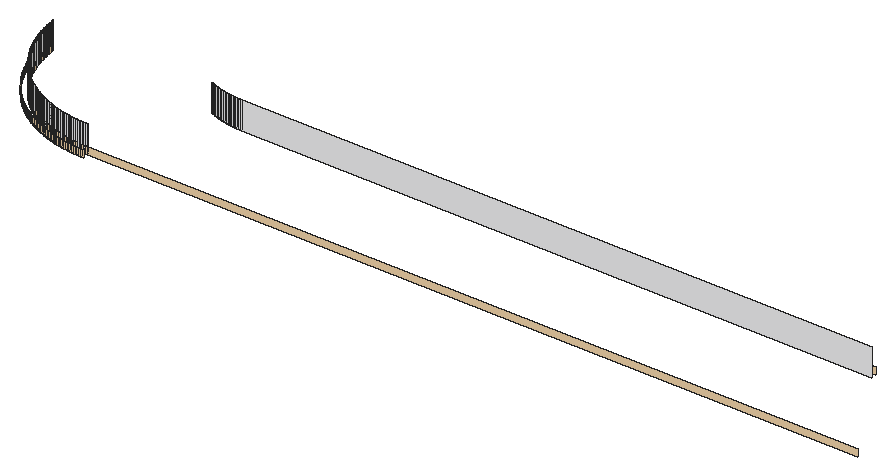
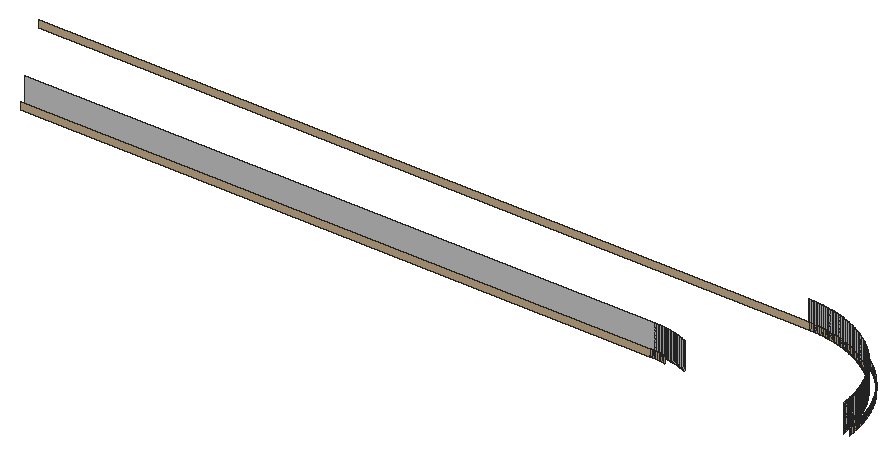
# SketchUp Ruby script. Lengths in inches.
U = 1.inch
M = Sketchup.active_model
def pt(a) = Geom::Point3d.new(a.map { |v| v * U })
def face(e, loops, mat)
  f = e.add_face(loops[0].map { |a| pt(a) })
  loops[1..].each { |l| e.add_face(l.map { |a| pt(a) }).erase! }
  f.material = f.back_material = mat if mat
  f
end
# faces: each face lists its corners as indices into pts; further lists are holes
def faces(e, pts, list, mat = nil) = list.each { |f| face(e, (f[0].is_a?(Array) ? f : [f]).map { |l| l.map { |i| pts[i] } }, mat) }
# xy, xz, yz: faces in a plane at the given z, y or x. An outline is a flat list of corners, or four numbers for a rectangle; further outlines are holes
def ring(l) = l.size == 4 ? [[l[0], l[1]], [l[2], l[1]], [l[2], l[3]], [l[0], l[3]]] : l.each_slice(2).to_a
def flat(e, list, mat, &to3) = list.each { |f| face(e, (f[0].is_a?(Array) ? f : [f]).map { |l| ring(l).map { |u, v| to3.(u, v) } }, mat) }
def xy(e, z, list, mat = nil) = flat(e, list, mat) { |x, y| [x, y, z] }
def xz(e, y, list, mat = nil) = flat(e, list, mat) { |x, z| [x, y, z] }
def yz(e, x, list, mat = nil) = flat(e, list, mat) { |y, z| [x, y, z] }
def lines(e, pts, list) = list.each { |a, b| e.add_line(pt(pts[a]), pt(pts[b])) }
# prism: a flat outline (further loops are holes) pulled along v
def prism(e, loops, v, mat = nil)
  f = face(e, loops, mat); d = Geom::Vector3d.new(v.map { |x| x * U })
  f.pushpull(f.normal.samedirection?(d) ? d.length : -d.length)
end
def box(e, o, s, mat = nil) = prism(e, [[o, [o[0] + s[0], o[1], o[2]], [o[0] + s[0], o[1] + s[1], o[2]], [o[0], o[1] + s[1], o[2]]]], [0, 0, s[2]], mat)
def at(x, y, z, deg = 0) = Geom::Transformation.translation(pt([x, y, z])) * Geom::Transformation.rotation(ORIGIN, Z_AXIS, deg.degrees)
def axes(o, x, y, z) = Geom::Transformation.new([*x, 0, *y, 0, *z, 0, *pt(o).to_a, 1])
def part(name) = M.definitions.add(name)
# library, detail: a bought-in or finely detailed component or shape, given as its bounding box
def library(name, o, s) = part(name).tap { |d| box(d.entities, o, s) }
def detail(e, o, s) = box(e.add_group.entities, o, s)
def put(e, d, t, mat = nil) = e.add_instance(d, t).tap { |i| i.material = mat if mat }
def group(e, t, mat = nil) = e.add_group.tap { |g| g.transformation = t; g.material = mat if mat }.entities
root = M.entities
M.materials.add("False Ceiling Light").color = [254, 223, 179]
M.materials.add("[Quartz Light Grey]").color = [251, 251, 252]
xz(root,43.5,[[44.53,115.32,44.76,116.49],[44.76,115.32,45,116.49]],"False Ceiling Light")
xz(root,44.5,[[44.55,115.32,44.77,116.49],[44.77,115.32,45.01,116.49],[45.01,115.32,176.99,116.49]],"False Ceiling Light")
xz(root,44.5,[[44.55,115.32,44.77,120],[44.77,115.32,45.01,120]],"[Quartz Light Grey]")
xz(root,62.5,[[56.8,115.32,56.99,120],[56.99,115.32,165.01,120]],"[Quartz Light Grey]")
xz(root,62.51,[[56.39,115.32,56.59,120]],"[Quartz Light Grey]")
xz(root,63.5,[[56.62,115.32,56.81,116.49],[56.81,115.32,56.99,116.49],[56.99,115.32,165.01,116.49]],"False Ceiling Light")
p = [[43.35,43.56,115.32],[43.59,43.54,115.32],[43.59,43.54,116.49],[43.35,43.56,116.49],[43.82,43.53,115.32],[43.82,43.53,116.49],
  [44.06,43.52,115.32],[44.06,43.52,116.49],[44.29,43.51,115.32],[44.29,43.51,116.49],[44.53,43.5,115.32],[44.53,43.5,116.49],
  [42.18,43.68,115.32],[42.41,43.65,115.32],[42.41,43.65,116.49],[42.18,43.68,116.49],[42.65,43.625,115.32],[42.65,43.625,116.49],
  [42.88,43.6,115.32],[42.88,43.6,116.49],[43.12,43.58,115.32],[43.12,43.58,116.49],[41.48,43.78,115.32],[41.71,43.74,115.32],
  [41.71,43.74,116.49],[41.48,43.78,116.49],[41.95,43.71,115.32],[41.95,43.71,116.49],[41.02,43.86,115.32],[41.25,43.82,115.32],
  [41.25,43.82,116.49],[41.02,43.86,116.49],[40.32,43.99,115.32],[40.55,43.94,115.32],[40.55,43.94,116.49],[40.32,43.99,116.49],
  [40.78,43.9,115.32],[40.78,43.9,116.49],[39.86,44.09,115.32],[40.09,44.04,115.32],[40.09,44.04,116.49],[39.86,44.09,116.49],
  [39.4,44.21,115.32],[39.63,44.15,115.32],[39.63,44.15,116.49],[39.4,44.21,116.49],[39.18,44.27,115.32],[39.18,44.27,116.49],
  [38.72,44.39,115.32],[38.95,44.33,115.32],[38.95,44.33,116.49],[38.72,44.39,116.49],[38.5,44.46,115.32],[38.5,44.46,116.49],
  [38.05,44.6,115.32],[38.27,44.53,115.32],[38.27,44.53,116.49],[38.05,44.6,116.49],[43.65,44.54,115.32],[43.43,44.56,115.32],
  [43.43,44.56,116.49],[43.65,44.54,116.49],[43.43,44.56,115.32],[43.65,44.54,115.32],[43.65,44.54,120],[43.43,44.56,120],
  [43.875,44.53,115.32],[43.875,44.53,116.49],[43.875,44.53,115.32],[43.875,44.53,120],[44.1,44.52,115.32],[44.1,44.52,116.49],
  [44.1,44.52,115.32],[44.1,44.52,120],[44.32,44.51,115.32],[44.32,44.51,116.49],[44.32,44.51,115.32],[44.32,44.51,120],
  [44.55,44.5,115.32],[44.55,44.5,116.49],[44.55,44.5,115.32],[44.55,44.5,120],[37.82,44.68,115.32],[37.82,44.68,116.49],
  [42.53,44.64,115.32],[42.31,44.67,115.32],[42.31,44.67,116.49],[42.53,44.64,116.49],[42.31,44.67,115.32],[42.53,44.64,115.32],
  [42.53,44.64,120],[42.31,44.67,120],[42.75,44.62,115.32],[42.75,44.62,116.49],[42.75,44.62,115.32],[42.75,44.62,120],
  [42.98,44.6,115.32],[42.98,44.6,116.49],[42.98,44.6,115.32],[42.98,44.6,120],[43.2,44.58,115.32],[43.2,44.58,116.49],
  [43.2,44.58,115.32],[43.2,44.58,120],[37.6,44.75,115.32],[37.6,44.75,116.49],[41.86,44.73,115.32],[41.64,44.76,115.32],
  [41.64,44.76,116.49],[41.86,44.73,116.49],[41.64,44.76,115.32],[41.86,44.73,115.32],[41.86,44.73,120],[41.64,44.76,120],
  [42.08,44.7,115.32],[42.08,44.7,116.49],[42.08,44.7,115.32],[42.08,44.7,120],[37.16,44.91,115.32],[37.38,44.83,115.32],
  [37.38,44.83,116.49],[37.16,44.91,116.49],[41.19,44.84,115.32],[40.97,44.88,115.32],[40.97,44.88,116.49],[41.19,44.84,116.49],
  [40.97,44.88,115.32],[41.19,44.84,115.32],[41.19,44.84,120],[40.97,44.88,120],[41.41,44.8,115.32],[41.41,44.8,116.49],
  [41.41,44.8,115.32],[41.41,44.8,120],[36.9375,44.99,115.32],[36.9375,44.99,116.49],[40.75,44.92,115.32],[40.53,44.97,115.32],
  [40.53,44.97,116.49],[40.75,44.92,116.49],[40.53,44.97,115.32],[40.75,44.92,115.32],[40.75,44.92,120],[40.53,44.97,120],
  [36.72,45.08,115.32],[36.72,45.08,116.49],[40.31,45.02,115.32],[40.09,45.07,115.32],[40.09,45.07,116.49],[40.31,45.02,116.49],
  [40.09,45.07,115.32],[40.31,45.02,115.32],[40.31,45.02,120],[40.09,45.07,120],[36.5,45.17,115.32],[36.5,45.17,116.49],
  [39.87,45.12,115.32],[39.65,45.18,115.32],[39.65,45.18,116.49],[39.87,45.12,116.49],[39.65,45.18,115.32],[39.87,45.12,115.32],
  [39.87,45.12,120],[39.65,45.18,120],[36.28,45.26,115.32],[36.28,45.26,116.49],[39.44,45.23,115.32],[39.22,45.29,115.32],
  [39.22,45.29,116.49],[39.44,45.23,116.49],[39.22,45.29,115.32],[39.44,45.23,115.32],[39.44,45.23,120],[39.22,45.29,120],
  [36.0625,45.35,115.32],[36.0625,45.35,116.49],[39,45.35,115.32],[39,45.35,116.49],[39,45.35,115.32],[39,45.35,120],
  [35.63,45.54,115.32],[35.85,45.45,115.32],[35.85,45.45,116.49],[35.63,45.54,116.49],[38.79,45.42,115.32],[38.57,45.48,115.32],
  [38.57,45.48,116.49],[38.79,45.42,116.49],[38.57,45.48,115.32],[38.79,45.42,115.32],[38.79,45.42,120],[38.57,45.48,120],
  [35.42,45.64,115.32],[35.42,45.64,116.49],[38.36,45.55,115.32],[38.36,45.55,116.49],[38.36,45.55,115.32],[38.36,45.55,120],
  [35.21,45.74,115.32],[35.21,45.74,116.49],[38.14,45.625,115.32],[37.93,45.7,115.32],[37.93,45.7,116.49],[38.14,45.625,116.49],
  [37.93,45.7,115.32],[38.14,45.625,115.32],[38.14,45.625,120],[37.93,45.7,120],[35,45.85,115.32],[35,45.85,116.49],
  [37.72,45.77,115.32],[37.72,45.77,116.49],[37.72,45.77,115.32],[37.72,45.77,120],[34.79,45.95,115.32],[34.79,45.95,116.49],
  [37.51,45.85,115.32],[37.3,45.93,115.32],[37.3,45.93,116.49],[37.51,45.85,116.49],[37.3,45.93,115.32],[37.51,45.85,115.32],
  [37.51,45.85,120],[37.3,45.93,120],[37.09,46.01,115.32],[37.09,46.01,116.49],[37.09,46.01,115.32],[37.09,46.01,120],
  [34.58,46.06,115.32],[34.58,46.06,116.49],[36.875,46.09,115.32],[36.875,46.09,116.49],[36.875,46.09,115.32],[36.875,46.09,120],
  [34.37,46.17,115.32],[34.37,46.17,116.49],[36.67,46.18,115.32],[36.67,46.18,116.49],[36.67,46.18,115.32],[36.67,46.18,120],
  [34.16,46.28,115.32],[34.16,46.28,116.49],[36.46,46.27,115.32],[36.46,46.27,116.49],[36.46,46.27,115.32],[36.46,46.27,120],
  [33.95,46.4,115.32],[33.95,46.4,116.49],[36.26,46.36,115.32],[36.26,46.36,116.49],[36.26,46.36,115.32],[36.26,46.36,120],
  [33.75,46.51,115.32],[33.75,46.51,116.49],[36.05,46.45,115.32],[36.05,46.45,116.49],[36.05,46.45,115.32],[36.05,46.45,120],
  [33.55,46.63,115.32],[33.55,46.63,116.49],[35.85,46.55,115.32],[35.64,46.64,115.32],[35.64,46.64,116.49],[35.85,46.55,116.49],
  [35.64,46.64,115.32],[35.85,46.55,115.32],[35.85,46.55,120],[35.64,46.64,120],[33.34,46.75,115.32],[33.34,46.75,116.49],
  [35.44,46.74,115.32],[35.44,46.74,116.49],[35.44,46.74,115.32],[35.44,46.74,120],[35.24,46.84,115.32],[35.24,46.84,116.49],
  [35.24,46.84,115.32],[35.24,46.84,120],[33.14,46.88,115.32],[33.14,46.88,116.49],[35.04,46.95,115.32],[35.04,46.95,116.49],
  [35.04,46.95,115.32],[35.04,46.95,120],[32.94,47,115.32],[32.94,47,116.49],[34.84,47.05,115.32],[34.84,47.05,116.49],
  [34.84,47.05,115.32],[34.84,47.05,120],[32.75,47.13,115.32],[32.75,47.13,116.49],[32.55,47.26,115.32],[32.55,47.26,116.49],
  [34.64,47.16,115.32],[34.64,47.16,116.49],[34.64,47.16,115.32],[34.64,47.16,120],[34.45,47.27,115.32],[34.45,47.27,116.49],
  [34.45,47.27,115.32],[34.45,47.27,120],[32.35,47.39,115.32],[32.35,47.39,116.49],[34.25,47.38,115.32],[34.25,47.38,116.49],
  [34.25,47.38,115.32],[34.25,47.38,120],[32.16,47.52,115.32],[32.16,47.52,116.49],[34.06,47.49,115.32],[34.06,47.49,116.49],
  [34.06,47.49,115.32],[34.06,47.49,120],[31.97,47.66,115.32],[31.97,47.66,116.49],[33.86,47.61,115.32],[33.86,47.61,116.49],
  [33.86,47.61,115.32],[33.86,47.61,120],[33.67,47.73,115.32],[33.67,47.73,116.49],[33.67,47.73,115.32],[33.67,47.73,120],
  [31.77,47.8,115.32],[31.77,47.8,116.49],[33.48,47.85,115.32],[33.48,47.85,116.49],[33.48,47.85,115.32],[33.48,47.85,120],
  [31.58,47.9375,115.32],[31.58,47.9375,116.49],[33.29,47.97,115.32],[33.29,47.97,116.49],[33.29,47.97,115.32],[33.29,47.97,120],
  [31.4,48.08,115.32],[31.4,48.08,116.49],[33.1,48.09,115.32],[33.1,48.09,116.49],[33.1,48.09,115.32],[33.1,48.09,120],
  [31.21,48.22,115.32],[31.21,48.22,116.49],[32.92,48.22,115.32],[32.92,48.22,116.49],[32.92,48.22,115.32],[32.92,48.22,120],
  [31.02,48.37,115.32],[31.02,48.37,116.49],[32.73,48.35,115.32],[32.73,48.35,116.49],[32.73,48.35,115.32],[32.73,48.35,120],
  [32.55,48.47,115.32],[32.55,48.47,116.49],[32.55,48.47,115.32],[32.55,48.47,120],[30.84,48.51,115.32],[30.84,48.51,116.49],
  [30.66,48.66,115.32],[30.66,48.66,116.49],[32.36,48.61,115.32],[32.36,48.61,116.49],[32.36,48.61,115.32],[32.36,48.61,120],
  [32.18,48.74,115.32],[32.18,48.74,116.49],[32.18,48.74,115.32],[32.18,48.74,120],[30.48,48.81,115.32],[30.48,48.81,116.49],
  [32,48.875,115.32],[32,48.875,116.49],[32,48.875,115.32],[32,48.875,120],[30.3,48.97,115.32],[30.3,48.97,116.49],
  [31.82,49.01,115.32],[31.82,49.01,116.49],[31.82,49.01,115.32],[31.82,49.01,120],[30.12,49.12,115.32],[30.12,49.12,116.49],
  [31.65,49.15,115.32],[31.65,49.15,116.49],[31.65,49.15,115.32],[31.65,49.15,120],[29.94,49.28,115.32],[29.94,49.28,116.49],
  [31.47,49.29,115.32],[31.47,49.29,116.49],[31.47,49.29,115.32],[31.47,49.29,120],[29.77,49.4375,115.32],[29.77,49.4375,116.49],
  [31.3,49.43,115.32],[31.3,49.43,116.49],[31.3,49.43,115.32],[31.3,49.43,120],[29.6,49.6,115.32],[29.6,49.6,116.49],
  [31.12,49.58,115.32],[31.12,49.58,116.49],[31.12,49.58,115.32],[31.12,49.58,120],[29.43,49.76,115.32],[29.43,49.76,116.49],
  [30.95,49.72,115.32],[30.95,49.72,116.49],[30.95,49.72,115.32],[30.95,49.72,120],[30.78,49.87,115.32],[30.78,49.87,116.49],
  [30.78,49.87,115.32],[30.78,49.87,120],[29.26,49.92,115.32],[29.26,49.92,116.49],[29.09,50.09,115.32],[29.09,50.09,116.49],
  [30.61,50.02,115.32],[30.61,50.02,116.49],[30.61,50.02,115.32],[30.61,50.02,120],[30.45,50.17,115.32],[30.45,50.17,116.49],
  [30.45,50.17,115.32],[30.45,50.17,120],[28.92,50.26,115.32],[28.92,50.26,116.49],[30.28,50.33,115.32],[30.28,50.33,116.49],
  [30.28,50.33,115.32],[30.28,50.33,120],[28.76,50.43,115.32],[28.76,50.43,116.49],[30.12,50.48,115.32],[30.12,50.48,116.49],
  [30.12,50.48,115.32],[30.12,50.48,120],[28.6,50.6,115.32],[28.6,50.6,116.49],[29.96,50.64,115.32],[29.96,50.64,116.49],
  [29.96,50.64,115.32],[29.96,50.64,120],[28.4375,50.77,115.32],[28.4375,50.77,116.49],[29.8,50.8,115.32],[29.8,50.8,116.49],
  [29.8,50.8,115.32],[29.8,50.8,120],[28.28,50.94,115.32],[28.28,50.94,116.49],[29.64,50.96,115.32],[29.64,50.96,116.49],
  [29.64,50.96,115.32],[29.64,50.96,120],[28.12,51.12,115.32],[28.12,51.12,116.49],[29.48,51.12,115.32],[29.48,51.12,116.49],
  [29.48,51.12,115.32],[29.48,51.12,120],[27.97,51.3,115.32],[27.97,51.3,116.49],[29.33,51.28,115.32],[29.33,51.28,116.49],
  [29.33,51.28,115.32],[29.33,51.28,120],[27.81,51.48,115.32],[27.81,51.48,116.49],[29.17,51.45,115.32],[29.17,51.45,116.49],
  [29.17,51.45,115.32],[29.17,51.45,120],[29.02,51.61,115.32],[29.02,51.61,116.49],[29.02,51.61,115.32],[29.02,51.61,120],
  [27.66,51.66,115.32],[27.66,51.66,116.49],[28.87,51.78,115.32],[28.87,51.78,116.49],[28.87,51.78,115.32],[28.87,51.78,120],
  [27.51,51.84,115.32],[27.51,51.84,116.49],[27.37,52.02,115.32],[27.37,52.02,116.49],[28.72,51.95,115.32],[28.72,51.95,116.49],
  [28.72,51.95,115.32],[28.72,51.95,120],[27.22,52.21,115.32],[27.22,52.21,116.49],[28.58,52.12,115.32],[28.58,52.12,116.49],
  [28.58,52.12,115.32],[28.58,52.12,120],[28.43,52.3,115.32],[28.43,52.3,116.49],[28.43,52.3,115.32],[28.43,52.3,120],
  [27.08,52.4,115.32],[27.08,52.4,116.49],[28.29,52.47,115.32],[28.29,52.47,116.49],[28.29,52.47,115.32],[28.29,52.47,120],
  [26.9375,52.58,115.32],[26.9375,52.58,116.49],[28.15,52.65,115.32],[28.15,52.65,116.49],[28.15,52.65,115.32],[28.15,52.65,120],
  [26.8,52.77,115.32],[26.8,52.77,116.49],[28.01,52.82,115.32],[28.01,52.82,116.49],[28.01,52.82,115.32],[28.01,52.82,120],
  [26.66,52.97,115.32],[26.66,52.97,116.49],[27.875,53,115.32],[27.875,53,116.49],[27.875,53,115.32],[27.875,53,120],
  [26.52,53.16,115.32],[26.52,53.16,116.49],[27.74,53.18,115.32],[27.74,53.18,116.49],[27.74,53.18,115.32],[27.74,53.18,120],
  [26.39,53.35,115.32],[26.39,53.35,116.49],[27.61,53.36,115.32],[27.61,53.36,116.49],[27.61,53.36,115.32],[27.61,53.36,120],
  [26.26,53.55,115.32],[26.26,53.55,116.49],[27.47,53.55,115.32],[27.47,53.55,116.49],[27.47,53.55,115.32],[27.47,53.55,120],
  [26.13,53.75,115.32],[26.13,53.75,116.49],[27.35,53.73,115.32],[27.35,53.73,116.49],[27.35,53.73,115.32],[27.35,53.73,120],
  [26,53.94,115.32],[26,53.94,116.49],[27.22,53.92,115.32],[27.22,53.92,116.49],[27.22,53.92,115.32],[27.22,53.92,120],
  [25.88,54.14,115.32],[25.88,54.14,116.49],[27.09,54.1,115.32],[27.09,54.1,116.49],[27.09,54.1,115.32],[27.09,54.1,120],
  [25.75,54.34,115.32],[25.75,54.34,116.49],[26.97,54.29,115.32],[26.97,54.29,116.49],[26.97,54.29,115.32],[26.97,54.29,120],
  [25.63,54.55,115.32],[25.63,54.55,116.49],[26.85,54.48,115.32],[26.85,54.48,116.49],[26.85,54.48,115.32],[26.85,54.48,120],
  [25.51,54.75,115.32],[25.51,54.75,116.49],[26.73,54.67,115.32],[26.73,54.67,116.49],[26.73,54.67,115.32],[26.73,54.67,120],
  [26.61,54.86,115.32],[26.61,54.86,116.49],[26.61,54.86,115.32],[26.61,54.86,120],[25.4,54.95,115.32],[25.4,54.95,116.49],
  [26.49,55.06,115.32],[26.49,55.06,116.49],[26.49,55.06,115.32],[26.49,55.06,120],[25.28,55.16,115.32],[25.28,55.16,116.49],
  [26.38,55.25,115.32],[26.38,55.25,116.49],[26.38,55.25,115.32],[26.38,55.25,120],[25.17,55.37,115.32],[25.17,55.37,116.49],
  [26.27,55.45,115.32],[26.27,55.45,116.49],[26.27,55.45,115.32],[26.27,55.45,120],[25.06,55.58,115.32],[25.06,55.58,116.49],
  [26.16,55.64,115.32],[26.16,55.64,116.49],[26.16,55.64,115.32],[26.16,55.64,120],[24.95,55.79,115.32],[24.95,55.79,116.49],
  [26.05,55.84,115.32],[26.05,55.84,116.49],[26.05,55.84,115.32],[26.05,55.84,120],[24.85,56,115.32],[24.85,56,116.49],
  [25.95,56.04,115.32],[25.95,56.04,116.49],[25.95,56.04,115.32],[25.95,56.04,120],[24.74,56.21,115.32],[24.74,56.21,116.49],
  [25.84,56.24,115.32],[25.84,56.24,116.49],[25.84,56.24,115.32],[25.84,56.24,120],[24.64,56.42,115.32],[24.64,56.42,116.49],
  [25.74,56.44,115.32],[25.74,56.44,116.49],[25.74,56.44,115.32],[25.74,56.44,120],[24.54,56.63,115.32],[24.54,56.63,116.49],
  [25.64,56.64,115.32],[25.64,56.64,116.49],[25.64,56.64,115.32],[25.64,56.64,120],[24.45,56.85,115.32],[24.45,56.85,116.49],
  [25.55,56.85,115.32],[25.55,56.85,116.49],[25.55,56.85,115.32],[25.55,56.85,120],[24.35,57.0625,115.32],[24.35,57.0625,116.49],
  [25.45,57.05,115.32],[25.45,57.05,116.49],[25.45,57.05,115.32],[25.45,57.05,120],[25.36,57.26,115.32],[25.36,57.26,116.49],
  [25.36,57.26,115.32],[25.36,57.26,120],[24.26,57.28,115.32],[24.26,57.28,116.49],[24.17,57.5,115.32],[24.17,57.5,116.49],
  [25.27,57.46,115.32],[25.27,57.46,116.49],[25.27,57.46,115.32],[25.27,57.46,120],[24.08,57.72,115.32],[24.08,57.72,116.49],
  [25.18,57.67,115.32],[25.18,57.67,116.49],[25.18,57.67,115.32],[25.18,57.67,120],[23.99,57.9375,115.32],[23.99,57.9375,116.49],
  [25.09,57.875,115.32],[25.09,57.875,116.49],[25.09,57.875,115.32],[25.09,57.875,120],[23.91,58.16,115.32],[23.91,58.16,116.49],
  [25.01,58.09,115.32],[25.01,58.09,116.49],[25.01,58.09,115.32],[25.01,58.09,120],[24.93,58.3,115.32],[24.93,58.3,116.49],
  [24.93,58.3,115.32],[24.93,58.3,120],[23.83,58.38,115.32],[23.83,58.38,116.49],[24.85,58.51,115.32],[24.85,58.51,116.49],
  [24.85,58.51,115.32],[24.85,58.51,120],[23.75,58.6,115.32],[23.75,58.6,116.49],[24.77,58.72,115.32],[24.77,58.72,116.49],
  [24.77,58.72,115.32],[24.77,58.72,120],[23.68,58.82,115.32],[23.68,58.82,116.49],[24.7,58.93,115.32],[24.7,58.93,116.49],
  [24.7,58.93,115.32],[24.7,58.93,120],[23.6,59.05,115.32],[23.6,59.05,116.49],[24.625,59.14,115.32],[24.625,59.14,116.49],
  [24.625,59.14,115.32],[24.625,59.14,120],[23.53,59.27,115.32],[23.53,59.27,116.49],[24.55,59.36,115.32],[24.55,59.36,116.49],
  [24.55,59.36,115.32],[24.55,59.36,120],[23.46,59.5,115.32],[23.46,59.5,116.49],[24.48,59.57,115.32],[24.48,59.57,116.49],
  [24.48,59.57,115.32],[24.48,59.57,120],[23.39,59.72,115.32],[23.39,59.72,116.49],[24.42,59.79,115.32],[24.42,59.79,116.49],
  [24.42,59.79,115.32],[24.42,59.79,120],[23.33,59.95,115.32],[23.33,59.95,116.49],[24.35,60,115.32],[24.35,60,116.49],
  [24.35,60,115.32],[24.35,60,120],[23.27,60.18,115.32],[23.27,60.18,116.49],[24.29,60.22,115.32],[24.29,60.22,116.49],
  [24.29,60.22,115.32],[24.29,60.22,120],[23.21,60.4,115.32],[23.21,60.4,116.49],[24.23,60.44,115.32],[24.23,60.44,116.49],
  [24.23,60.44,115.32],[24.23,60.44,120],[23.15,60.63,115.32],[23.15,60.63,116.49],[24.18,60.65,115.32],[24.18,60.65,116.49],
  [24.18,60.65,115.32],[24.18,60.65,120],[23.09,60.86,115.32],[23.09,60.86,116.49],[24.12,60.87,115.32],[24.12,60.87,116.49],
  [24.12,60.87,115.32],[24.12,60.87,120],[23.04,61.09,115.32],[23.04,61.09,116.49],[24.07,61.09,115.32],[24.07,61.09,116.49],
  [24.07,61.09,115.32],[24.07,61.09,120],[22.99,61.32,115.32],[22.99,61.32,116.49],[24.02,61.31,115.32],[24.02,61.31,116.49],
  [24.02,61.31,115.32],[24.02,61.31,120],[22.94,61.55,115.32],[22.94,61.55,116.49],[23.97,61.53,115.32],[23.97,61.53,116.49],
  [23.97,61.53,115.32],[23.97,61.53,120],[23.92,61.75,115.32],[23.92,61.75,116.49],[23.92,61.75,115.32],[23.92,61.75,120],
  [22.9,61.78,115.32],[22.9,61.78,116.49],[22.86,62.02,115.32],[22.86,62.02,116.49],[23.88,61.97,115.32],[23.88,61.97,116.49],
  [23.88,61.97,115.32],[23.88,61.97,120],[22.82,62.25,115.32],[22.82,62.25,116.49],[23.84,62.19,115.32],[23.84,62.19,116.49],
  [23.84,62.19,115.32],[23.84,62.19,120],[22.78,62.48,115.32],[22.78,62.48,116.49],[23.8,62.41,115.32],[23.8,62.41,116.49],
  [23.8,62.41,115.32],[23.8,62.41,120],[23.76,62.64,115.32],[23.76,62.64,116.49],[23.76,62.64,115.32],[23.76,62.64,120],
  [22.74,62.71,115.32],[22.74,62.71,116.49],[55.78,62.55,115.32],[55.58,62.57,115.32],[55.58,62.57,120],[55.78,62.55,120],
  [55.98,62.53,115.32],[55.98,62.53,120],[56.1875,62.52,115.32],[56.1875,62.52,120],[56.39,62.51,115.32],[56.39,62.51,120],
  [56.8,62.5,115.32],[56.59,62.51,115.32],[56.59,62.51,120],[56.8,62.5,120],[23.73,62.86,115.32],[23.73,62.86,116.49],
  [23.73,62.86,115.32],[23.73,62.86,120],[54.97,62.63,115.32],[54.77,62.66,115.32],[54.77,62.66,120],[54.97,62.63,120],
  [55.17,62.61,115.32],[55.17,62.61,120],[55.375,62.59,115.32],[55.375,62.59,120],[22.71,62.95,115.32],[22.71,62.95,116.49],
  [54.37,62.73,115.32],[54.17,62.76,115.32],[54.17,62.76,120],[54.37,62.73,120],[54.57,62.69,115.32],[54.57,62.69,120],
  [53.77,62.84,115.32],[53.57,62.88,115.32],[53.57,62.88,120],[53.77,62.84,120],[53.97,62.8,115.32],[53.97,62.8,120],
  [22.68,63.18,115.32],[22.68,63.18,116.49],[23.7,63.08,115.32],[23.7,63.08,116.49],[23.7,63.08,115.32],[23.7,63.08,120],
  [53.37,62.93,115.32],[53.17,62.98,115.32],[53.17,62.98,120],[53.37,62.93,120],[52.98,63.03,115.32],[52.78,63.09,115.32],
  [52.78,63.09,120],[52.98,63.03,120],[23.67,63.31,115.32],[23.67,63.31,116.49],[23.67,63.31,115.32],[23.67,63.31,120],
  [52.58,63.14,115.32],[52.39,63.2,115.32],[52.39,63.2,120],[52.58,63.14,120],[22.65,63.41,115.32],[22.65,63.41,116.49],
  [52.19,63.26,115.32],[52.19,63.26,120],[23.64,63.53,115.32],[23.64,63.53,116.49],[23.64,63.53,115.32],[23.64,63.53,120],
  [52,63.33,115.32],[51.81,63.39,115.32],[51.81,63.39,120],[52,63.33,120],[22.625,63.65,115.32],[22.625,63.65,116.49],
  [51.62,63.46,115.32],[51.62,63.46,120],[23.62,63.75,115.32],[23.62,63.75,116.49],[23.62,63.75,115.32],[23.62,63.75,120],
  [51.43,63.54,115.32],[51.24,63.61,115.32],[51.24,63.61,120],[51.43,63.54,120],[55.67,63.5625,115.32],[55.86,63.54,115.32],
  [55.86,63.54,116.49],[55.67,63.5625,116.49],[56.05,63.53,115.32],[56.05,63.53,116.49],[56.24,63.52,115.32],[56.24,63.52,116.49],
  [56.43,63.51,115.32],[56.43,63.51,116.49],[56.62,63.5,115.32],[56.62,63.5,116.49],[51.05,63.6875,115.32],[51.05,63.6875,120],
  [54.91,63.65,115.32],[55.1,63.625,115.32],[55.1,63.625,116.49],[54.91,63.65,116.49],[55.29,63.6,115.32],[55.29,63.6,116.49],
  [55.48,63.58,115.32],[55.48,63.58,116.49],[50.86,63.77,115.32],[50.86,63.77,120],[54.16,63.78,115.32],[54.35,63.74,115.32],
  [54.35,63.74,116.49],[54.16,63.78,116.49],[54.54,63.71,115.32],[54.54,63.71,116.49],[54.72,63.68,115.32],[54.72,63.68,116.49]]
faces(root,p,[[0,1,2,3],[1,4,5,2],[4,6,7,5],[6,8,9,7],[8,10,11,9],[12,13,14,15],[13,16,17,14],[16,18,19,17],
  [18,20,21,19],[20,0,3,21],[22,23,24,25],[23,26,27,24],[26,12,15,27],[28,29,30,31],[29,22,25,30],[32,33,34,35],
  [33,36,37,34],[36,28,31,37],[38,39,40,41],[39,32,35,40],[42,43,44,45],[43,38,41,44],[46,42,45,47],[48,49,50,51],
  [49,46,47,50],[52,48,51,53],[54,55,56,57],[55,52,53,56],[58,59,60,61],[66,58,61,67],[70,66,67,71],[74,70,71,75],
  [78,74,75,79],[82,54,57,83],[84,85,86,87],[92,84,87,93],[96,92,93,97],[100,96,97,101],[59,100,101,60],[104,82,83,105],
  [106,107,108,109],[114,106,109,115],[85,114,115,86],[118,119,120,121],[119,104,105,120],[122,123,124,125],[130,122,125,131],[107,130,131,108],
  [134,118,121,135],[136,137,138,139],[123,136,139,124],[144,134,135,145],[146,147,148,149],[137,146,149,138],[154,144,145,155],[156,157,158,159],
  [147,156,159,148],[164,154,155,165],[166,167,168,169],[157,166,169,158],[174,164,165,175],[167,176,177,168],[180,181,182,183],[181,174,175,182],
  [184,185,186,187],[176,184,187,177],[192,180,183,193],[185,194,195,186],[198,192,193,199],[200,201,202,203],[194,200,203,195],[208,198,199,209],
  [201,210,211,202],[214,208,209,215],[216,217,218,219],[210,216,219,211],[217,224,225,218],[228,214,215,229],[224,230,231,225],[234,228,229,235],
  [230,236,237,231],[240,234,235,241],[236,242,243,237],[246,240,241,247],[242,248,249,243],[252,246,247,253],[248,254,255,249],[258,252,253,259],
  [260,261,262,263],[254,260,263,255],[268,258,259,269],[261,270,271,262],[270,274,275,271],[278,268,269,279],[274,280,281,275],[284,278,279,285],
  [280,286,287,281],[290,284,285,291],[292,290,291,293],[286,294,295,287],[294,298,299,295],[302,292,293,303],[298,304,305,299],[308,302,303,309],
  [304,310,311,305],[314,308,309,315],[310,316,317,311],[316,320,321,317],[324,314,315,325],[320,326,327,321],[330,324,325,331],[326,332,333,327],
  [336,330,331,337],[332,338,339,333],[342,336,337,343],[338,344,345,339],[348,342,343,349],[344,350,351,345],[350,354,355,351],[358,348,349,359],
  [360,358,359,361],[354,362,363,355],[362,366,367,363],[370,360,361,371],[366,372,373,367],[376,370,371,377],[372,378,379,373],[382,376,377,383],
  [378,384,385,379],[388,382,383,389],[384,390,391,385],[394,388,389,395],[390,396,397,391],[400,394,395,401],[396,402,403,397],[406,400,401,407],
  [402,408,409,403],[408,412,413,409],[416,406,407,417],[418,416,417,419],[412,420,421,413],[420,424,425,421],[428,418,419,429],[424,430,431,425],
  [434,428,429,435],[430,436,437,431],[440,434,435,441],[436,442,443,437],[446,440,441,447],[442,448,449,443],[452,446,447,453],[448,454,455,449],
  [458,452,453,459],[454,460,461,455],[464,458,459,465],[460,466,467,461],[470,464,465,471],[466,472,473,467],[472,476,477,473],[480,470,471,481],
  [476,482,483,477],[486,480,481,487],[488,486,487,489],[482,490,491,483],[494,488,489,495],[490,496,497,491],[496,500,501,497],[504,494,495,505],
  [500,506,507,501],[510,504,505,511],[506,512,513,507],[516,510,511,517],[512,518,519,513],[522,516,517,523],[518,524,525,519],[528,522,523,529],
  [524,530,531,525],[534,528,529,535],[530,536,537,531],[540,534,535,541],[536,542,543,537],[546,540,541,547],[542,548,549,543],[552,546,547,553],
  [548,554,555,549],[558,552,553,559],[554,560,561,555],[564,558,559,565],[560,566,567,561],[570,564,565,571],[566,572,573,567],[576,570,571,577],
  [572,578,579,573],[578,582,583,579],[586,576,577,587],[582,588,589,583],[592,586,587,593],[588,594,595,589],[598,592,593,599],[594,600,601,595],
  [604,598,599,605],[600,606,607,601],[610,604,605,611],[606,612,613,607],[616,610,611,617],[612,618,619,613],[622,616,617,623],[618,624,625,619],
  [628,622,623,629],[624,630,631,625],[634,628,629,635],[630,636,637,631],[640,634,635,641],[636,642,643,637],[646,640,641,647],[642,648,649,643],
  [648,652,653,649],[656,646,647,657],[658,656,657,659],[652,660,661,653],[664,658,659,665],[660,666,667,661],[670,664,665,671],[666,672,673,667],
  [676,670,671,677],[672,678,679,673],[678,682,683,679],[686,676,677,687],[682,688,689,683],[692,686,687,693],[688,694,695,689],[698,692,693,699],
  [694,700,701,695],[704,698,699,705],[700,706,707,701],[710,704,705,711],[706,712,713,707],[716,710,711,717],[712,718,719,713],[722,716,717,723],
  [718,724,725,719],[728,722,723,729],[724,730,731,725],[734,728,729,735],[730,736,737,731],[740,734,735,741],[736,742,743,737],[746,740,741,747],
  [742,748,749,743],[752,746,747,753],[748,754,755,749],[758,752,753,759],[754,760,761,755],[764,758,759,765],[760,766,767,761],[770,764,765,771],
  [766,772,773,767],[772,776,777,773],[780,770,771,781],[782,780,781,783],[776,784,785,777],[788,782,783,789],[784,790,791,785],[794,788,789,795],
  [790,796,797,791],[796,800,801,797],[804,794,795,805],[800,820,821,801],[832,804,805,833],[846,832,833,847],[820,848,849,821],[848,860,861,849],
  [868,846,847,869],[860,872,873,861],[880,868,869,881],[872,884,885,873],[892,893,894,895],[893,896,897,894],[896,898,899,897],[898,900,901,899],
  [900,902,903,901],[906,907,908,909],[907,910,911,908],[910,912,913,911],[912,892,895,913],[916,917,918,919],[917,920,921,918],[920,922,923,921],
  [922,906,909,923]],"False Ceiling Light")
faces(root,p,[[62,63,64,65],[63,68,69,64],[68,72,73,69],[72,76,77,73],[76,80,81,77],[88,89,90,91],[89,94,95,90],[94,98,99,95],
  [98,102,103,99],[102,62,65,103],[110,111,112,113],[111,116,117,112],[116,88,91,117],[126,127,128,129],[127,132,133,128],[132,110,113,133],
  [140,141,142,143],[141,126,129,142],[150,151,152,153],[151,140,143,152],[160,161,162,163],[161,150,153,162],[170,171,172,173],[171,160,163,172],
  [178,170,173,179],[188,189,190,191],[189,178,179,190],[196,188,191,197],[204,205,206,207],[205,196,197,206],[212,204,207,213],[220,221,222,223],
  [221,212,213,222],[226,220,223,227],[232,226,227,233],[238,232,233,239],[244,238,239,245],[250,244,245,251],[256,250,251,257],[264,265,266,267],
  [265,256,257,266],[272,264,267,273],[276,272,273,277],[282,276,277,283],[288,282,283,289],[296,288,289,297],[300,296,297,301],[306,300,301,307],
  [312,306,307,313],[318,312,313,319],[322,318,319,323],[328,322,323,329],[334,328,329,335],[340,334,335,341],[346,340,341,347],[352,346,347,353],
  [356,352,353,357],[364,356,357,365],[368,364,365,369],[374,368,369,375],[380,374,375,381],[386,380,381,387],[392,386,387,393],[398,392,393,399],
  [404,398,399,405],[410,404,405,411],[414,410,411,415],[422,414,415,423],[426,422,423,427],[432,426,427,433],[438,432,433,439],[444,438,439,445],
  [450,444,445,451],[456,450,451,457],[462,456,457,463],[468,462,463,469],[474,468,469,475],[478,474,475,479],[484,478,479,485],[492,484,485,493],
  [498,492,493,499],[502,498,499,503],[508,502,503,509],[514,508,509,515],[520,514,515,521],[526,520,521,527],[532,526,527,533],[538,532,533,539],
  [544,538,539,545],[550,544,545,551],[556,550,551,557],[562,556,557,563],[568,562,563,569],[574,568,569,575],[580,574,575,581],[584,580,581,585],
  [590,584,585,591],[596,590,591,597],[602,596,597,603],[608,602,603,609],[614,608,609,615],[620,614,615,621],[626,620,621,627],[632,626,627,633],
  [638,632,633,639],[644,638,639,645],[650,644,645,651],[654,650,651,655],[662,654,655,663],[668,662,663,669],[674,668,669,675],[680,674,675,681],
  [684,680,681,685],[690,684,685,691],[696,690,691,697],[702,696,697,703],[708,702,703,709],[714,708,709,715],[720,714,715,721],[726,720,721,727],
  [732,726,727,733],[738,732,733,739],[744,738,739,745],[750,744,745,751],[756,750,751,757],[762,756,757,763],[768,762,763,769],[774,768,769,775],
  [778,774,775,779],[786,778,779,787],[792,786,787,793],[798,792,793,799],[802,798,799,803],[806,807,808,809],[810,806,809,811],[812,810,811,813],
  [814,812,813,815],[816,817,818,819],[822,802,803,823],[824,825,826,827],[828,824,827,829],[830,828,829,831],[807,830,831,808],[834,835,836,837],
  [838,834,837,839],[825,838,839,826],[840,841,842,843],[844,840,843,845],[835,844,845,836],[850,822,823,851],[852,853,854,855],[841,852,855,842],
  [856,857,858,859],[853,856,859,854],[862,850,851,863],[864,865,866,867],[857,864,867,858],[865,870,871,866],[874,862,863,875],[876,877,878,879],
  [870,876,879,871],[877,882,883,878],[886,874,875,887],[888,889,890,891],[882,888,891,883],[889,904,905,890],[904,914,915,905]],"[Quartz Light Grey]")
